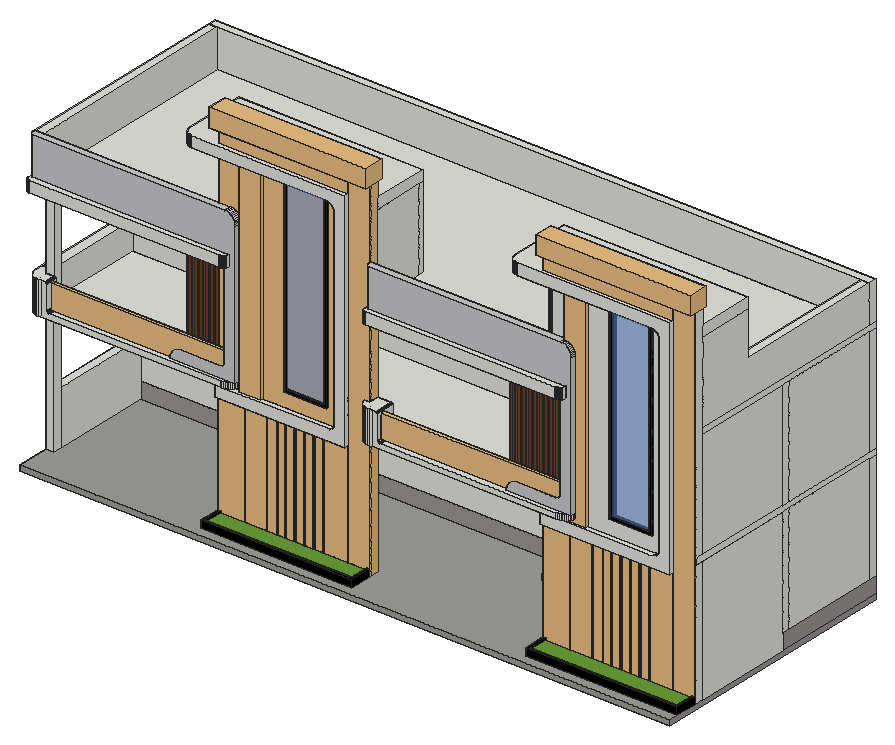
# SketchUp Ruby script. Lengths in inches.
U = 1.inch
M = Sketchup.active_model
def pt(a) = Geom::Point3d.new(a.map { |v| v * U })
def face(e, loops, mat)
  f = e.add_face(loops[0].map { |a| pt(a) })
  loops[1..].each { |l| e.add_face(l.map { |a| pt(a) }).erase! }
  f.material = f.back_material = mat if mat
  f
end
# faces: each face lists its corners as indices into pts; further lists are holes
def faces(e, pts, list, mat = nil) = list.each { |f| face(e, (f[0].is_a?(Array) ? f : [f]).map { |l| l.map { |i| pts[i] } }, mat) }
# xy, xz, yz: faces in a plane at the given z, y or x. An outline is a flat list of corners, or four numbers for a rectangle; further outlines are holes
def ring(l) = l.size == 4 ? [[l[0], l[1]], [l[2], l[1]], [l[2], l[3]], [l[0], l[3]]] : l.each_slice(2).to_a
def flat(e, list, mat, &to3) = list.each { |f| face(e, (f[0].is_a?(Array) ? f : [f]).map { |l| ring(l).map { |u, v| to3.(u, v) } }, mat) }
def xy(e, z, list, mat = nil) = flat(e, list, mat) { |x, y| [x, y, z] }
def xz(e, y, list, mat = nil) = flat(e, list, mat) { |x, z| [x, y, z] }
def yz(e, x, list, mat = nil) = flat(e, list, mat) { |y, z| [x, y, z] }
def lines(e, pts, list) = list.each { |a, b| e.add_line(pt(pts[a]), pt(pts[b])) }
# prism: a flat outline (further loops are holes) pulled along v
def prism(e, loops, v, mat = nil)
  f = face(e, loops, mat); d = Geom::Vector3d.new(v.map { |x| x * U })
  f.pushpull(f.normal.samedirection?(d) ? d.length : -d.length)
end
def box(e, o, s, mat = nil) = prism(e, [[o, [o[0] + s[0], o[1], o[2]], [o[0] + s[0], o[1] + s[1], o[2]], [o[0], o[1] + s[1], o[2]]]], [0, 0, s[2]], mat)
def at(x, y, z, deg = 0) = Geom::Transformation.translation(pt([x, y, z])) * Geom::Transformation.rotation(ORIGIN, Z_AXIS, deg.degrees)
def axes(o, x, y, z) = Geom::Transformation.new([*x, 0, *y, 0, *z, 0, *pt(o).to_a, 1])
def part(name) = M.definitions.add(name)
# library, detail: a bought-in or finely detailed component or shape, given as its bounding box
def library(name, o, s) = part(name).tap { |d| box(d.entities, o, s) }
def detail(e, o, s) = box(e.add_group.entities, o, s)
def put(e, d, t, mat = nil) = e.add_instance(d, t).tap { |i| i.material = mat if mat }
def group(e, t, mat = nil) = e.add_group.tap { |g| g.transformation = t; g.material = mat if mat }.entities
root = M.entities
M.materials.add("[Color M09]").color = [0, 0, 0]
M.materials.add("[Concrete Aggregate Smoke]").color = [154, 150, 148]
M.materials.add("[Concrete Block 8x8 Gray]").color = [157, 158, 154]
M.materials.add("[Grass Dark Green]").color = [106, 157, 55]
M.materials.add("[Polished Concrete New]").color = [200, 200, 203]
M.materials.add("[Translucent Glass Blue]").color = [100, 149, 237]
M.materials["[Translucent Glass Blue]"].alpha = 0.5
M.materials.add("[Wood Bamboo]").color = [177, 105, 43]
M.materials.add("[Wood Cherry Original]").color = [152, 86, 42]
M.materials.add("[Wood Veneer 01]").color = [120, 70, 37]
c1 = part("Group\#3")
prism(c1.entities,[[[0,3,60],[60,3,60],[60,3,0],[0,3,0]],[[27,3,3],[27,3,57],[3,3,57],[3,3,3]],[[33,3,57],[33,3,3],[57,3,3],[57,3,57]]],[0,-3,0])
c2 = part("Group\#4")
xz(c2.entities,0,[[0,0,24,54]])
c3 = part("Group\#5")
xz(c3.entities,0,[[0,0,24,54]])
c4 = part("Group\#6")
prism(c4.entities,[[[60,3,0],[0,3,0],[0,3,60],[60,3,60]],[[57,3,57],[33,3,57],[33,3,3],[57,3,3]],[[3,3,57],[3,3,3],[27,3,3],[27,3,57]]],[0,-3,0])
c5 = part("Group\#7")
xz(c5.entities,0,[[0,0,24,54]])
c6 = part("Group\#8")
xz(c6.entities,0,[[0,0,24,54]])
c7 = part("Group\#9")
prism(c7.entities,[[[3,6,93],[3,6,0],[0,6,0],[0,6,96],[48,6,96],[48,6,0],[45,6,0],[45,6,93]]],[0,-6,0])
c8 = part("Group\#10")
box(c8.entities,[0,0,0],[42,2,93])
c9 = part("Group\#11")
prism(c9.entities,[[[0,1,0.8],[0,1,0],[0,0,0],[0,0,41.3125],[0,1,41.3125],[0,1,40.7],[0,0.3,40.7],[0,0.3,0.8]]],[1.5,0,0])
c10 = part("Group\#12")
prism(c10.entities,[[[3,6,93],[3,6,0],[0,6,0],[0,6,96],[48,6,96],[48,6,0],[45,6,0],[45,6,93]]],[0,-6,0])
c11 = part("Group\#13")
box(c11.entities,[0,0,0],[42,2,93])
c12 = part("Group\#14")
prism(c12.entities,[[[0,1.5,1.15],[0,1.5,0],[0,0,0],[0,0,13.6875],[0,1.5,13.6875],[0,1.5,12.73],[0,0.52,12.73],[0,0.52,1.15]]],[1.4375,0,0])
c13 = part("Group\#16")
box(c13.entities,[0,0,0],[9,111,120])
c14 = part("Group\#17")
box(c14.entities,[0,0,0],[9,111,120])
c15 = library("Group\#20",[0,0,0],[168,9,390])
c16 = library("Group\#22",[0,0,0],[24,2,390])
c17 = library("Group\#23",[0,0,0],[24,2,390])
c18 = part("Group\#30")
box(c18.entities,[0,0,0],[2,1,122])
c19 = part("Group\#31")
put(c19.entities,c18,at(15,0,0))
put(c19.entities,c18,at(48,0,0))
put(c19.entities,c18,at(3,0,0))
put(c19.entities,c18,at(12,0,0))
put(c19.entities,c18,at(33,0,0))
put(c19.entities,c18,at(51,0,0))
put(c19.entities,c18,at(54,0,0))
put(c19.entities,c18,at(39,0,0))
put(c19.entities,c18,at(9,0,0))
put(c19.entities,c18,at(24,0,0))
put(c19.entities,c18,at(18,0,0))
put(c19.entities,c18,at(21,0,0))
put(c19.entities,c18,at(36,0,0))
put(c19.entities,c18,at(30,0,0))
put(c19.entities,c18,at(27,0,0))
put(c19.entities,c18,at(45,0,0))
put(c19.entities,c18,at(42,0,0))
put(c19.entities,c18,at(57,0,0))
put(c19.entities,c18,at(0,0,0))
put(c19.entities,c18,at(6,0,0))
put(c19.entities,c18,at(69,0,0))
put(c19.entities,c18,at(66,0,0))
put(c19.entities,c18,at(63,0,0))
put(c19.entities,c18,at(60,0,0))
c20 = library("Group\#32",[0,0,0],[114,2,122])
c21 = library("Group\#36",[0,0,0],[114,2,122])
c22 = library("Group\#33",[0,0,0],[30,2,122])
c23 = library("Group\#61",[0,0,0],[30,2,122])
c24 = library("Group\#66",[0,0,0],[24,3,226])
c25 = library("Group\#34",[-0.2,0,0],[24.2,3,226])
c26 = library("Group\#44",[0,0,0],[192.84,3.98,26.63])
c27 = library("Group\#62",[0,0,0],[192.84,3.98,26.63])
c28 = library("Group\#52",[-2,0,0],[137,2,18])
c29 = part("Group\#53")
prism(c29.entities,[[[0,33,18],[0,33,0],[0,0,0],[0,0,6],[0,11,6],[0,11,12],[0,22,12],[0,22,18]]],[48,0,0])
c30 = library("Group\#54",[-10.44,-4.48,0],[173.22,22.01,20])
c31 = library("Group\#58",[-9.83,-3.875,0],[172,20.8,20])
c32 = part("Group\#59")
box(c32.entities,[0,0,0],[2.6875,5.375,120])
c33 = part("Group\#60")
put(c33.entities,c32,at(12,0,0))
put(c33.entities,c32,at(0,0,0))
put(c33.entities,c32,at(36,0,0))
put(c33.entities,c32,at(54,0,0))
put(c33.entities,c32,at(48,0,0))
put(c33.entities,c32,at(30,0,0))
put(c33.entities,c32,at(6,0,0))
put(c33.entities,c32,at(24,0,0))
put(c33.entities,c32,at(18,0,0))
put(c33.entities,c32,at(42,0,0))
c34 = part("Group\#65")
xy(c34.entities,0,[[0,0,168,24]])
xy(c34.entities,6.3125,[[3,3,165,24]],"[Grass Dark Green]")
xy(c34.entities,8,[[0,0,168,0,168,24,165,24,165,3,3,3,3,24,0,24]])
xz(c34.entities,0,[[0,0,168,8]])
xz(c34.entities,3,[[3,6.3125,165,8]])
xz(c34.entities,24,[[0,0,0,8,3,8,3,6.3125,165,6.3125,165,8,168,8,168,0]])
yz(c34.entities,0,[[0,0,24,8]])
yz(c34.entities,3,[[3,6.3125,24,8]])
yz(c34.entities,165,[[3,6.3125,24,8]])
yz(c34.entities,168,[[0,0,24,8]])
box(root,[276.07,44.3,150],[48,0.7,210])
box(root,[636.07,44.4,150],[48,0.6,210])
xy(root,138,[[590.07,35,600.07,35,588.38,35.84]])
p = [[586.19,36,138],[588.38,35.84,138],[588.07,36,138],[366.35,34,138],[366.35,34,174],[372.07,34,174],
  [372.07,45,174],[215.75,27.83,270],[221.82,27.83,270],[221.82,27.83,257.98],[593.94,27.83,270],[588.07,27.83,270],
  [593.94,27.83,258.125],[593.94,27.83,257.98],[588.07,27.83,257.98],[207.03,39.48,360],[206.71,40.1,360],[206.39,40.72,360],
  [206.07,41.34,360],[205.74,41.95,360],[205.41,42.5625,360],[205.08,43.18,360],[204.74,43.79,360],[204.07,45,360],
  [204.41,44.39,360],[207.34,38.86,360],[207.65,38.24,360],[207.96,37.61,360]]
lines(root,p,[[0,1],[1,2],[3,4],[4,5],[5,6],[7,8],[8,9],[10,11],[10,12],[12,13],[13,14],[15,16],
  [16,17],[17,18],[18,19],[19,20],[20,21],[21,22],[23,24],[24,22],[15,25],[25,26],[26,27]])
g1 = group(root,at(12.07,45,6),"[Concrete Aggregate Smoke]")
xy(g1,-12,[[0,-45,720,240]])
xy(g1,-6,[[0,111,720,240]])
xy(g1,-6,[[0,-45,720,111]],"[Concrete Block 8x8 Gray]")
xy(g1,12,[[0,111,720,240]])
xz(g1,-45,[[0,-12,720,-6]],"[Concrete Block 8x8 Gray]")
xz(g1,111,[[0,-6,720,12]])
xz(g1,240,[[0,-12,720,-6],[0,-6,720,12]])
yz(g1,0,[[-45,-12,240,-6],[111,-6,240,12]])
yz(g1,720,[[-45,-12,240,-6],[111,-6,240,12]])
g2 = group(root,at(12.07,156,18))
prism(g2,[[[720,9,0],[528,9,0],[528,9,96],[480,9,96],[480,9,0],[180,9,0],[180,9,96],[132,9,96],[132,9,0],[0,9,0],[0,9,120],[720,9,120]],[[36,9,96],[36,9,36],[96,9,36],[96,9,96]],[[444,9,36],[444,9,96],[384,9,96],[384,9,36]]],[0,-9,0])
put(root,c1,at(48.07,156,54),"[Wood Veneer 01]")
put(root,c2,at(81.07,156,57),"[Translucent Glass Blue]")
put(root,c3,at(51.07,156,57),"[Translucent Glass Blue]")
put(root,c4,at(396.07,156,54),"[Wood Veneer 01]")
put(root,c5,at(429.07,156,57),"[Translucent Glass Blue]")
put(root,c6,at(399.07,156,57),"[Translucent Glass Blue]")
put(root,c7,at(144.07,156,18),"[Wood Bamboo]")
put(root,c8,at(147.07,159,18),"[Wood Bamboo]")
put(root,c9,at(151.76,158,35.81),"[Wood Bamboo]")
put(root,c10,at(492.07,156,18),"[Wood Bamboo]")
put(root,c11,at(495.07,159,18),"[Wood Bamboo]")
put(root,c12,at(497.5625,157.5,63.91),"[Wood Bamboo]")
g3 = group(root,at(12.07,276,18))
box(g3,[0,0,0],[720,9,120])
put(root,c13,at(12.07,165,18))
put(root,c14,at(723.07,165,18))
put(root,c8,at(147.07,159,144),"[Wood Bamboo]")
g4 = group(root,at(12.07,276,144))
box(g4,[-11.67,0,0],[731.67,9,120])
put(root,c12,at(497.5625,157.5,189.91),"[Wood Bamboo]")
put(root,c7,at(144.07,156,144),"[Wood Bamboo]")
put(root,c1,at(48.07,156,180),"[Wood Veneer 01]")
put(root,c13,at(0.39,165,144))
put(root,c11,at(495.07,159,144),"[Wood Bamboo]")
put(root,c2,at(81.07,156,183),"[Translucent Glass Blue]")
put(root,c5,at(429.07,156,183),"[Translucent Glass Blue]")
put(root,c3,at(51.07,156,183),"[Translucent Glass Blue]")
put(root,c4,at(396.07,156,180),"[Wood Veneer 01]")
put(root,c6,at(399.07,156,183),"[Translucent Glass Blue]")
put(root,c14,at(723.07,165,144))
put(root,c10,at(492.07,156,144),"[Wood Bamboo]")
g5 = group(root,at(12.07,156,144))
prism(g5,[[[720,9,0],[528,9,0],[528,9,96],[480,9,96],[480,9,0],[180,9,0],[180,9,96],[132,9,96],[132,9,0],[-11.67,9,0],[-11.67,9,120],[720,9,120]],[[36,9,96],[36,9,36],[96,9,36],[96,9,96]],[[444,9,36],[444,9,96],[384,9,96],[384,9,36]]],[0,-9,0])
put(root,c9,at(151.76,158,161.81),"[Wood Bamboo]")
g6 = group(root,at(12.07,156,138))
prism(g6,[[[720,129,0],[720,-119.45,0],[9,-119.45,0],[9,-111,0],[-11.67,-111,0],[-11.67,0,0],[-11.67,129,0]]],[0,0,6])
g7 = group(root,at(12.07,36,0))
prism(g7,[[[9,0,0],[9,9,0],[9,9,264],[9,0.55,264],[9,0.55,138],[9,0,138]]],[-9,0,0])
put(root,c15,at(204.07,36,0))
g8 = group(root,at(564.07,36,0))
xy(g8,0,[[0,0,168,9]])
xy(g8,138,[[0,0,22.125,9]])
xy(g8,150,[[72,0,120,9]])
xy(g8,264,[[9,0,7.83,0.08,6.67,0.31,5.56,0.69,4.5,1.21,3.52,1.86,2.64,2.64,1.86,3.52,1.21,4.5,0.69,5.56,0.31,6.67,0.08,7.83,0,9,22.125,9,22.125,0]])
xy(g8,360,[[72,0,120,9]])
xy(g8,390,[[9,0,168,0,168,9,0,9,0.08,7.83,0.31,6.67,0.69,5.56,1.21,4.5,1.86,3.52,2.64,2.64,3.52,1.86,4.5,1.21,5.56,0.69,6.67,0.31,7.83,0.08]])
xz(g8,0,[[[0,0,168,0,168,390,9,390,9,264,22.125,264,22.125,138,0,138],[72,150,120,360]]])
xz(g8,9,[[[0,0,0,138,22.125,138,22.125,264,0,264,0,390,168,390,168,0],[72,150,120,360]]])
yz(g8,0,[[0,0,9,138]])
yz(g8,22.125,[[0,138,9,264]])
yz(g8,72,[[0,150,9,360]])
yz(g8,120,[[0,150,9,360]])
yz(g8,168,[[0,0,9,390]])
p = [[9,0,390],[7.83,0.08,390],[7.83,0.08,264],[9,0,264],[6.67,0.31,390],[6.67,0.31,264],
  [5.56,0.69,390],[5.56,0.69,264],[4.5,1.21,390],[4.5,1.21,264],[3.52,1.86,390],[3.52,1.86,264],
  [2.64,2.64,390],[2.64,2.64,264],[1.86,3.52,390],[1.86,3.52,264],[1.21,4.5,390],[1.21,4.5,264],
  [0.69,5.56,390],[0.69,5.56,264],[0.31,6.67,390],[0.31,6.67,264],[0.08,7.83,390],[0.08,7.83,264],
  [0,9,390],[0,9,264]]
faces(g8,p,[[0,1,2,3],[1,4,5,2],[4,6,7,5],[6,8,9,7],[8,10,11,9],[10,12,13,11],[12,14,15,13],[14,16,17,15],
  [16,18,19,17],[18,20,21,19],[20,22,23,21],[22,24,25,23]])
put(root,c16,at(348.07,34,0),"[Polished Concrete New]")
put(root,c17,at(708.07,34,0),"[Polished Concrete New]")
g9 = group(root,at(204.07,30,122))
xy(g9,0,[[0,0,144,6]])
xy(g9,12,[[11.49,0,126.92,6]])
xy(g9,16,[[0,0,11.49,6]])
xy(g9,238,[[-25.46,0,-26.83,0.09,-28.1875,0.36,-29.49,0.8,-30.73,1.41,-31.875,2.18,-32.91,3.09,-33.82,4.125,-34.59,5.27,-35.2,6.51,-35.64,7.8125,-35.91,9.17,-36,10.54,-36,78,168,78,168,15,3.89,15,3.89,6,122.55,6,122.55,0]])
xy(g9,250,[[-25.46,0,144,0,144,6,3.89,6,3.89,15,168,15,168,78,-36,78,-36,10.54,-35.91,9.17,-35.64,7.8125,-35.2,6.51,-34.59,5.27,-33.82,4.125,-32.91,3.09,-31.875,2.18,-30.73,1.41,-29.49,0.8,-28.1875,0.36,-26.83,0.09]])
xz(g9,0,[[0,0,144,0,144,250,-25.46,250,-25.46,238,122.55,238,123.78,237.92,124.99,237.68,126.17,237.28,127.27,236.73,128.3,236.05,129.23,235.23,130.05,234.3,130.73,233.27,131.28,232.17,131.68,230.99,131.92,229.78,132,228.55,132,17.08,131.96,16.42,131.83,15.77,131.61,15.14,131.32,14.54,130.95,13.99,130.51,13.49,130.01,13.05,129.46,12.68,128.86,12.39,128.23,12.17,127.58,12.04,126.92,12,11.49,12,11.49,16,0,16]])
xz(g9,6,[[0,0,0,16,11.49,16,11.49,12,126.92,12,127.58,12.04,128.23,12.17,128.86,12.39,129.46,12.68,130.01,13.05,130.51,13.49,130.95,13.99,131.32,14.54,131.61,15.14,131.83,15.77,131.96,16.42,132,17.08,132,228.55,131.92,229.78,131.68,230.99,131.28,232.17,130.73,233.27,130.05,234.3,129.23,235.23,128.3,236.05,127.27,236.73,126.17,237.28,124.99,237.68,123.78,237.92,122.55,238,3.89,238,3.89,250,144,250,144,0]])
xz(g9,15,[[3.89,238,168,250]])
xz(g9,78,[[-36,238,168,250]])
yz(g9,-36,[[10.54,238,78,250]])
yz(g9,0,[[0,0,6,16]])
yz(g9,3.89,[[6,238,15,250]])
yz(g9,11.49,[[0,12,6,16]])
yz(g9,132,[[0,17.08,6,228.55]])
yz(g9,144,[[0,0,6,250]])
yz(g9,168,[[15,238,78,250]])
p = [[127.58,6,12.04],[126.92,6,12],[126.92,0,12],[127.58,0,12.04],[128.23,6,12.17],[128.23,0,12.17],
  [128.86,6,12.39],[128.86,0,12.39],[129.46,6,12.68],[129.46,0,12.68],[130.01,6,13.05],[130.01,0,13.05],
  [130.51,6,13.49],[130.51,0,13.49],[130.95,6,13.99],[130.95,0,13.99],[131.32,6,14.54],[131.32,0,14.54],
  [131.61,6,15.14],[131.61,0,15.14],[131.83,6,15.77],[131.83,0,15.77],[131.96,6,16.42],[131.96,0,16.42],
  [132,6,17.08],[132,0,17.08],[131.92,6,229.78],[132,6,228.55],[132,0,228.55],[131.92,0,229.78],
  [131.68,6,230.99],[131.68,0,230.99],[131.28,6,232.17],[131.28,0,232.17],[130.73,6,233.27],[130.73,0,233.27],
  [130.05,6,234.3],[130.05,0,234.3],[129.23,6,235.23],[129.23,0,235.23],[128.3,6,236.05],[128.3,0,236.05],
  [127.27,6,236.73],[127.27,0,236.73],[126.17,6,237.28],[126.17,0,237.28],[124.99,6,237.68],[124.99,0,237.68],
  [123.78,6,237.92],[123.78,0,237.92],[122.55,6,238],[122.55,0,238],[-25.46,0,250],[-26.83,0.09,250],
  [-26.83,0.09,238],[-25.46,0,238],[-28.1875,0.36,250],[-28.1875,0.36,238],[-29.49,0.8,250],[-29.49,0.8,238],
  [-30.73,1.41,250],[-30.73,1.41,238],[-31.875,2.18,250],[-31.875,2.18,238],[-32.91,3.09,250],[-32.91,3.09,238],
  [-33.82,4.125,250],[-33.82,4.125,238],[-34.59,5.27,250],[-34.59,5.27,238],[-35.2,6.51,250],[-35.2,6.51,238],
  [-35.64,7.8125,250],[-35.64,7.8125,238],[-35.91,9.17,250],[-35.91,9.17,238],[-36,10.54,250],[-36,10.54,238]]
faces(g9,p,[[0,1,2,3],[4,0,3,5],[6,4,5,7],[8,6,7,9],[10,8,9,11],[12,10,11,13],[14,12,13,15],[16,14,15,17],
  [18,16,17,19],[20,18,19,21],[22,20,21,23],[24,22,23,25],[26,27,28,29],[30,26,29,31],[32,30,31,33],[34,32,33,35],
  [36,34,35,37],[38,36,37,39],[40,38,39,41],[42,40,41,43],[44,42,43,45],[46,44,45,47],[48,46,47,49],[50,48,49,51],
  [52,53,54,55],[53,56,57,54],[56,58,59,57],[58,60,61,59],[60,62,63,61],[62,64,65,63],[64,66,67,65],[66,68,69,67],
  [68,70,71,69],[70,72,73,71],[72,74,75,73],[74,76,77,75]])
g10 = group(root,at(564.07,30,122))
xy(g10,0,[[0,0,144,6]])
xy(g10,12,[[11.8,0,124.1,6]])
xy(g10,16,[[0,0,11.8,6]])
xy(g10,238,[[-24.32,0,-25.84,0.1,-27.34,0.4,-28.79,0.89,-30.16,1.57,-31.43,2.41,-32.58,3.42,-33.59,4.57,-34.43,5.84,-35.11,7.21,-35.6,8.66,-35.9,10.16,-36,11.68,-36,78,168,78,168,15,2.79,15,2.79,6,123.21,6,123.21,0]])
xy(g10,250,[[-24.32,0,144,0,144,6,2.79,6,2.79,15,168,15,168,78,-36,78,-36,11.68,-35.9,10.16,-35.6,8.66,-35.11,7.21,-34.43,5.84,-33.59,4.57,-32.58,3.42,-31.43,2.41,-30.16,1.57,-28.79,0.89,-27.34,0.4,-25.84,0.1]])
xz(g10,0,[[0,0,144,0,144,250,-24.32,250,-24.32,238,123.21,238,124.36,237.92,125.49,237.7,126.58,237.33,127.61,236.82,128.5625,236.18,129.43,235.43,130.18,234.5625,130.82,233.61,131.33,232.58,131.7,231.49,131.92,230.36,132,229.21,132,19.9,131.93,18.87,131.73,17.86,131.4,16.88,130.94,15.95,130.37,15.09,129.6875,14.3125,128.91,13.63,128.05,13.06,127.12,12.6,126.14,12.27,125.13,12.07,124.1,12,11.8,12,11.8,16,0,16]])
xz(g10,6,[[0,0,0,16,11.8,16,11.8,12,124.1,12,125.13,12.07,126.14,12.27,127.12,12.6,128.05,13.06,128.91,13.63,129.6875,14.3125,130.37,15.09,130.94,15.95,131.4,16.88,131.73,17.86,131.93,18.87,132,19.9,132,229.21,131.92,230.36,131.7,231.49,131.33,232.58,130.82,233.61,130.18,234.5625,129.43,235.43,128.5625,236.18,127.61,236.82,126.58,237.33,125.49,237.7,124.36,237.92,123.21,238,2.79,238,2.79,250,144,250,144,0]])
xz(g10,15,[[2.79,238,168,250]])
xz(g10,78,[[-36,238,168,250]])
yz(g10,-36,[[11.68,238,78,250]])
yz(g10,0,[[0,0,6,16]])
yz(g10,2.79,[[6,238,15,250]])
yz(g10,11.8,[[0,12,6,16]])
yz(g10,132,[[0,19.9,6,229.21]])
yz(g10,144,[[0,0,6,250]])
yz(g10,168,[[15,238,78,250]])
p = [[125.13,6,12.07],[124.1,6,12],[124.1,0,12],[125.13,0,12.07],[126.14,6,12.27],[126.14,0,12.27],
  [127.12,6,12.6],[127.12,0,12.6],[128.05,6,13.06],[128.05,0,13.06],[128.91,6,13.63],[128.91,0,13.63],
  [129.6875,6,14.3125],[129.6875,0,14.3125],[130.37,6,15.09],[130.37,0,15.09],[130.94,6,15.95],[130.94,0,15.95],
  [131.4,6,16.88],[131.4,0,16.88],[131.73,6,17.86],[131.73,0,17.86],[131.93,6,18.87],[131.93,0,18.87],
  [132,6,19.9],[132,0,19.9],[131.92,6,230.36],[132,6,229.21],[132,0,229.21],[131.92,0,230.36],
  [131.7,6,231.49],[131.7,0,231.49],[131.33,6,232.58],[131.33,0,232.58],[130.82,6,233.61],[130.82,0,233.61],
  [130.18,6,234.5625],[130.18,0,234.5625],[129.43,6,235.43],[129.43,0,235.43],[128.5625,6,236.18],[128.5625,0,236.18],
  [127.61,6,236.82],[127.61,0,236.82],[126.58,6,237.33],[126.58,0,237.33],[125.49,6,237.7],[125.49,0,237.7],
  [124.36,6,237.92],[124.36,0,237.92],[123.21,6,238],[123.21,0,238],[-24.32,0,250],[-25.84,0.1,250],
  [-25.84,0.1,238],[-24.32,0,238],[-27.34,0.4,250],[-27.34,0.4,238],[-28.79,0.89,250],[-28.79,0.89,238],
  [-30.16,1.57,250],[-30.16,1.57,238],[-31.43,2.41,250],[-31.43,2.41,238],[-32.58,3.42,250],[-32.58,3.42,238],
  [-33.59,4.57,250],[-33.59,4.57,238],[-34.43,5.84,250],[-34.43,5.84,238],[-35.11,7.21,250],[-35.11,7.21,238],
  [-35.6,8.66,250],[-35.6,8.66,238],[-35.9,10.16,250],[-35.9,10.16,238],[-36,11.68,250],[-36,11.68,238]]
faces(g10,p,[[0,1,2,3],[4,0,3,5],[6,4,5,7],[8,6,7,9],[10,8,9,11],[12,10,11,13],[14,12,13,15],[16,14,15,17],
  [18,16,17,19],[20,18,19,21],[22,20,21,23],[24,22,23,25],[26,27,28,29],[30,26,29,31],[32,30,31,33],[34,32,33,35],
  [36,34,35,37],[38,36,37,39],[40,38,39,41],[42,40,41,43],[44,42,43,45],[46,44,45,47],[48,46,47,49],[50,48,49,51],
  [52,53,54,55],[53,56,57,54],[56,58,59,57],[58,60,61,59],[60,62,63,61],[62,64,65,63],[64,66,67,65],[66,68,69,67],
  [68,70,71,69],[70,72,73,71],[72,74,75,73],[74,76,77,75]])
g11 = group(root,at(276.07,35,150),"[Color M09]")
prism(g11,[[[0,4,0],[0,4,210],[48,4,210],[48,4,0]],[[45,4,207],[3,4,207],[3,4,3],[45,4,3]]],[0,-4,0])
g12 = group(root,at(279.07,36,153),"[Translucent Glass Blue]")
xz(g12,0,[[0,0,42,204]])
g13 = group(root,at(636.07,35,150))
prism(g13,[[[0,4,0],[0,4,210],[48,4,210],[48,4,0]],[[3,4,3],[45,4,3],[45,4,207],[3,4,207]]],[0,-4,0],"[Color M09]")
g14 = group(root,at(639.07,36,153),"[Translucent Glass Blue]")
xz(g14,0,[[0,0,42,204]])
put(root,c19,at(252.07,35,0),"[Wood Bamboo]")
put(root,c20,at(234.07,34,0))
put(root,c19,at(613.07,35,0),"[Wood Bamboo]")
put(root,c21,at(594.07,34,0))
put(root,c22,at(204.07,34,0))
put(root,c23,at(564.07,34,0))
put(root,c24,at(228.07,33,134),"[Wood Cherry Original]")
put(root,c25,at(588.07,33,134),"[Wood Cherry Original]")
g15 = group(root,at(16.39,24,138))
xy(g15,0,[[-3.89,-0.41,-5.81,-0.17,-7.67,0.37,-9.43,1.19,-11.05,2.28,-12.48,3.6,-12.88,4.09,-4.23,4.09,-4.2,3.61,-4.1,3.125,-3.93,2.66,-3.69,2.21,-3.4,1.79,-3.05,1.4,-2.64,1.05,-2.19,0.74,-1.7,0.48,-1.17,0.26,-0.625,0.1,-0.05,0,-1.96,-0.35],[-0.05,0,-0.625,0.1,-1.17,0.26,-1.7,0.48,-2.19,0.74,-2.64,1.05,-3.05,1.4,-3.4,1.79,-3.69,2.21,-3.93,2.66,-4.1,3.125,-4.2,3.61,-4.23,4.09,-12.88,4.09,-13.71,5.125,-14.69,6.82,-15.41,8.66,-15.85,10.58,-15.99,12.55,-15.99,21,-4.32,21,-4.32,12.55,211.68,12.55,211.68,10.85,211.57,9.4375,211.24,8.04,210.69,6.7,209.94,5.43,209,4.25,207.88,3.18,206.6,2.24,205.19,1.45,203.67,0.83,202.0625,0.37,200.4,0.09,198.7,0]])
xy(g15,6,[[9.74,0,198.7,0,200.4,0.09,202.0625,0.37,203.67,0.83,205.19,1.45,206.6,2.24,207.88,3.18,209,4.25,209.94,5.43,210.69,6.7,211.24,8.04,211.57,9.4375,211.68,10.85,211.68,12.55,9.74,12.55]])
xy(g15,36,[[-3.89,-0.41,-1.96,-0.35,-0.05,0,4.125,0,4.125,12.55,-4.32,12.55,-4.32,21,-15.99,21,-15.99,12.55,-15.85,10.58,-15.41,8.66,-14.69,6.82,-13.71,5.125,-12.88,4.09,-12.48,3.6,-11.05,2.28,-9.43,1.19,-7.67,0.37,-5.81,-0.17]])
xz(g15,0,[[-0.05,0,198.7,0,198.7,6,9.74,6,9.32,6.02,8.91,6.09,8.51,6.2,8.13,6.36,7.78,6.55,7.47,6.79,7.19,7.05,6.96,7.34,6.77,7.66,6.64,7.99,6.56,8.33,6.53,8.68,6.53,33.99,6.51,34.25,6.45,34.51,6.35,34.76,6.21,35,6.03,35.21,5.82,35.41,5.59,35.58,5.33,35.73,5.05,35.85,4.75,35.93,4.4375,35.98,4.125,36,-0.05,36]])
xz(g15,12.55,[[-4.32,0,-4.32,36,4.125,36,4.4375,35.98,4.75,35.93,5.05,35.85,5.33,35.73,5.59,35.58,5.82,35.41,6.03,35.21,6.21,35,6.35,34.76,6.45,34.51,6.51,34.25,6.53,33.99,6.53,8.68,6.56,8.33,6.64,7.99,6.77,7.66,6.96,7.34,7.19,7.05,7.47,6.79,7.78,6.55,8.13,6.36,8.51,6.2,8.91,6.09,9.32,6.02,9.74,6,211.68,6,211.68,0]])
xz(g15,21,[[-15.99,0,-4.32,36]])
yz(g15,-15.99,[[12.55,0,21,36]])
yz(g15,-4.32,[[12.55,0,21,36]])
yz(g15,6.53,[[0,8.68,12.55,33.99]])
yz(g15,211.68,[[10.85,0,12.55,6]])
p = [[-3.89,-0.41,36],[-5.81,-0.17,36],[-5.81,-0.17,0],[-3.89,-0.41,0],[-1.96,-0.35,36],[-1.96,-0.35,0],
  [-0.05,0,36],[-0.05,0,0],[-7.67,0.37,36],[-7.67,0.37,0],[200.4,0.09,6],[198.7,0,6],
  [198.7,0,0],[200.4,0.09,0],[202.0625,0.37,6],[202.0625,0.37,0],[-9.43,1.19,36],[-9.43,1.19,0],
  [203.67,0.83,6],[203.67,0.83,0],[205.19,1.45,6],[205.19,1.45,0],[-11.05,2.28,36],[-11.05,2.28,0],
  [206.6,2.24,6],[206.6,2.24,0],[207.88,3.18,6],[207.88,3.18,0],[-12.48,3.6,36],[-12.48,3.6,0],
  [209,4.25,6],[209,4.25,0],[-12.88,4.09,36],[-12.88,4.09,0],[-13.71,5.125,36],[-13.71,5.125,0],
  [209.94,5.43,6],[209.94,5.43,0],[-14.69,6.82,36],[-14.69,6.82,0],[210.69,6.7,6],[210.69,6.7,0],
  [211.24,8.04,6],[211.24,8.04,0],[-15.41,8.66,36],[-15.41,8.66,0],[211.57,9.4375,6],[211.57,9.4375,0],
  [-15.85,10.58,36],[-15.85,10.58,0],[211.68,10.85,6],[211.68,10.85,0],[-15.99,12.55,36],[-15.99,12.55,0],
  [9.32,12.55,6.02],[8.91,12.55,6.09],[8.91,0,6.09],[9.32,0,6.02],[9.74,12.55,6],[9.74,0,6],
  [8.51,12.55,6.2],[8.51,0,6.2],[8.13,12.55,6.36],[8.13,0,6.36],[7.78,12.55,6.55],[7.78,0,6.55],
  [7.47,12.55,6.79],[7.47,0,6.79],[7.19,12.55,7.05],[7.19,0,7.05],[6.96,12.55,7.34],[6.96,0,7.34],
  [6.77,12.55,7.66],[6.77,0,7.66],[6.64,12.55,7.99],[6.64,0,7.99],[6.56,12.55,8.33],[6.56,0,8.33],
  [6.53,12.55,8.68],[6.53,0,8.68],[6.53,12.55,33.99],[6.51,12.55,34.25],[6.51,0,34.25],[6.53,0,33.99],
  [6.45,12.55,34.51],[6.45,0,34.51],[6.35,12.55,34.76],[6.35,0,34.76],[6.21,12.55,35],[6.21,0,35],
  [6.03,12.55,35.21],[6.03,0,35.21],[5.82,12.55,35.41],[5.82,0,35.41],[5.59,12.55,35.58],[5.59,0,35.58],
  [5.33,12.55,35.73],[5.33,0,35.73],[5.05,12.55,35.85],[5.05,0,35.85],[4.75,12.55,35.93],[4.75,0,35.93],
  [4.4375,12.55,35.98],[4.4375,0,35.98],[4.125,12.55,36],[4.125,0,36],[-4.1,3.125,33.15],[-4.23,4.09,36],
  [-4.23,4.09,0]]
faces(g15,p,[[0,1,2,3],[4,0,3,5],[6,4,5,7],[1,8,9,2],[10,11,12,13],[14,10,13,15],[8,16,17,9],[18,14,15,19],
  [20,18,19,21],[16,22,23,17],[24,20,21,25],[26,24,25,27],[22,28,29,23],[30,26,27,31],[28,32,33,29],[32,34,35,33],
  [36,30,31,37],[34,38,39,35],[40,36,37,41],[42,40,41,43],[38,44,45,39],[46,42,43,47],[44,48,49,45],[50,46,47,51],
  [48,52,53,49],[54,55,56,57],[58,54,57,59],[55,60,61,56],[60,62,63,61],[62,64,65,63],[64,66,67,65],[66,68,69,67],
  [68,70,71,69],[70,72,73,71],[72,74,75,73],[74,76,77,75],[76,78,79,77],[80,81,82,83],[81,84,85,82],[84,86,87,85],
  [86,88,89,87],[88,90,91,89],[90,92,93,91],[92,94,95,93],[94,96,97,95],[96,98,99,97],[98,100,101,99],[100,102,103,101],
  [102,104,105,103]])
lines(g15,p,[[106,6],[107,108]])
g16 = group(root,at(382.51,24,138))
xy(g16,0,[[-4,-0.41,-5.97,-0.17,-7.89,0.37,-9.7,1.19,-11.36,2.28,-12.84,3.6,-13.25,4.09,-4.35,4.09,-4.32,3.61,-4.21,3.125,-4.04,2.66,-3.8,2.21,-3.5,1.79,-3.13,1.4,-2.72,1.05,-2.25,0.74,-1.75,0.48,-1.21,0.26,-0.64,0.1,-0.06,0,-2.01,-0.35],[-0.06,0,-0.64,0.1,-1.21,0.26,-1.75,0.48,-2.25,0.74,-2.72,1.05,-3.13,1.4,-3.5,1.79,-3.8,2.21,-4.04,2.66,-4.21,3.125,-4.32,3.61,-4.35,4.09,-13.25,4.09,-14.1,5.125,-15.11,6.82,-15.85,8.66,-16.3,10.58,-16.45,12.55,-16.45,21,217.73,21,217.73,10.85,217.61,9.4375,217.27,8.04,216.71,6.7,215.94,5.43,214.97,4.25,213.82,3.18,212.51,2.24,211.05,1.45,209.49,0.83,207.83,0.37,206.12,0.09,204.38,0]])
xy(g16,6,[[10.01,0,204.38,0,206.12,0.09,207.83,0.37,209.49,0.83,211.05,1.45,212.51,2.24,213.82,3.18,214.97,4.25,215.94,5.43,216.71,6.7,217.27,8.04,217.61,9.4375,217.73,10.85,217.73,21,10.01,21]])
xy(g16,36,[[-4,-0.41,-2.01,-0.35,-0.06,0,4.24,0,4.24,21,-16.45,21,-16.45,12.55,-16.3,10.58,-15.85,8.66,-15.11,6.82,-14.1,5.125,-13.25,4.09,-12.84,3.6,-11.36,2.28,-9.7,1.19,-7.89,0.37,-5.97,-0.17]])
xz(g16,0,[[-0.06,0,204.38,0,204.38,6,10.01,6,9.58,6.02,9.16,6.09,8.75,6.2,8.36,6.36,8.01,6.55,7.68,6.79,7.4,7.05,7.16,7.34,6.97,7.66,6.83,7.99,6.74,8.33,6.71,8.68,6.71,33.99,6.69,34.25,6.63,34.51,6.53,34.76,6.38,35,6.2,35.21,5.99,35.41,5.75,35.58,5.48,35.73,5.1875,35.85,4.88,35.93,4.57,35.98,4.24,36,-0.06,36]])
xz(g16,21,[[-16.45,0,-16.45,36,4.24,36,4.57,35.98,4.88,35.93,5.1875,35.85,5.48,35.73,5.75,35.58,5.99,35.41,6.2,35.21,6.38,35,6.53,34.76,6.63,34.51,6.69,34.25,6.71,33.99,6.71,8.68,6.74,8.33,6.83,7.99,6.97,7.66,7.16,7.34,7.4,7.05,7.68,6.79,8.01,6.55,8.36,6.36,8.75,6.2,9.16,6.09,9.58,6.02,10.01,6,217.73,6,217.73,0]])
yz(g16,-16.45,[[12.55,0,21,36]])
yz(g16,6.71,[[0,8.68,21,33.99]])
yz(g16,217.73,[[10.85,0,21,6]])
p = [[-4,-0.41,36],[-5.97,-0.17,36],[-5.97,-0.17,0],[-4,-0.41,0],[-2.01,-0.35,36],[-2.01,-0.35,0],
  [-0.06,0,36],[-0.06,0,0],[-7.89,0.37,36],[-7.89,0.37,0],[206.12,0.09,6],[204.38,0,6],
  [204.38,0,0],[206.12,0.09,0],[207.83,0.37,6],[207.83,0.37,0],[-9.7,1.19,36],[-9.7,1.19,0],
  [209.49,0.83,6],[209.49,0.83,0],[211.05,1.45,6],[211.05,1.45,0],[-11.36,2.28,36],[-11.36,2.28,0],
  [212.51,2.24,6],[212.51,2.24,0],[213.82,3.18,6],[213.82,3.18,0],[-12.84,3.6,36],[-12.84,3.6,0],
  [214.97,4.25,6],[214.97,4.25,0],[-13.25,4.09,36],[-13.25,4.09,0],[-14.1,5.125,36],[-14.1,5.125,0],
  [215.94,5.43,6],[215.94,5.43,0],[-15.11,6.82,36],[-15.11,6.82,0],[216.71,6.7,6],[216.71,6.7,0],
  [217.27,8.04,6],[217.27,8.04,0],[-15.85,8.66,36],[-15.85,8.66,0],[217.61,9.4375,6],[217.61,9.4375,0],
  [-16.3,10.58,36],[-16.3,10.58,0],[217.73,10.85,6],[217.73,10.85,0],[-16.45,12.55,36],[-16.45,12.55,0],
  [9.58,21,6.02],[9.16,21,6.09],[9.16,0,6.09],[9.58,0,6.02],[10.01,21,6],[10.01,0,6],
  [8.75,21,6.2],[8.75,0,6.2],[8.36,21,6.36],[8.36,0,6.36],[8.01,21,6.55],[8.01,0,6.55],
  [7.68,21,6.79],[7.68,0,6.79],[7.4,21,7.05],[7.4,0,7.05],[7.16,21,7.34],[7.16,0,7.34],
  [6.97,21,7.66],[6.97,0,7.66],[6.83,21,7.99],[6.83,0,7.99],[6.74,21,8.33],[6.74,0,8.33],
  [6.71,21,8.68],[6.71,0,8.68],[6.71,21,33.99],[6.69,21,34.25],[6.69,0,34.25],[6.71,0,33.99],
  [6.63,21,34.51],[6.63,0,34.51],[6.53,21,34.76],[6.53,0,34.76],[6.38,21,35],[6.38,0,35],
  [6.2,21,35.21],[6.2,0,35.21],[5.99,21,35.41],[5.99,0,35.41],[5.75,21,35.58],[5.75,0,35.58],
  [5.48,21,35.73],[5.48,0,35.73],[5.1875,21,35.85],[5.1875,0,35.85],[4.88,21,35.93],[4.88,0,35.93],
  [4.57,21,35.98],[4.57,0,35.98],[4.24,21,36],[4.24,0,36],[-4.21,3.125,33.15],[-4.35,4.09,36],
  [-4.35,4.09,0]]
faces(g16,p,[[0,1,2,3],[4,0,3,5],[6,4,5,7],[1,8,9,2],[10,11,12,13],[14,10,13,15],[8,16,17,9],[18,14,15,19],
  [20,18,19,21],[16,22,23,17],[24,20,21,25],[26,24,25,27],[22,28,29,23],[30,26,27,31],[28,32,33,29],[32,34,35,33],
  [36,30,31,37],[34,38,39,35],[40,36,37,41],[42,40,41,43],[38,44,45,39],[46,42,43,47],[44,48,49,45],[50,46,47,51],
  [48,52,53,49],[54,55,56,57],[58,54,57,59],[55,60,61,56],[60,62,63,61],[62,64,65,63],[64,66,67,65],[66,68,69,67],
  [68,70,71,69],[70,72,73,71],[72,74,75,73],[74,76,77,75],[76,78,79,77],[80,81,82,83],[81,84,85,82],[84,86,87,85],
  [86,88,89,87],[88,90,91,89],[90,92,93,91],[92,94,95,93],[94,96,97,95],[96,98,99,97],[98,100,101,99],[100,102,103,101],
  [102,104,105,103]])
lines(g16,p,[[106,6],[107,108]])
g17 = group(root,at(372.3125,27.83,144),"[Polished Concrete New]")
xy(g17,0,[[155.75,0,215.75,8.17],[215.75,0,217.75,8.17],[217.75,0,228,8.17]])
xy(g17,12,[[167.75,0,211.64,8.17]])
xy(g17,126,[[3.78,0,3.23,0.29,2.71,0.64,2.23,1.03,1.78,1.46,1.38,1.9375,1.02,2.45,0.72,2.99,0.46,3.56,0.26,4.15,0.12,4.75,0.03,5.37,0,5.99,0,8.17,215.75,8.17,215.75,0]])
xy(g17,168,[[3.78,0,215.75,0,215.75,8.17,0,8.17,0,5.99,0.03,5.37,0.12,4.75,0.26,4.15,0.46,3.56,0.72,2.99,1.02,2.45,1.38,1.9375,1.78,1.46,2.23,1.03,2.71,0.64,3.23,0.29]])
xz(g17,0,[[155.75,0,228,0,228,156,228.04,157.64,227.84,159.26,227.39,160.84,226.72,162.33,225.84,163.71,224.75,164.9375,223.5,165.99,222.11,166.85,220.6,167.49,219.02,167.9,217.39,168.07,215.75,168,3.78,168,3.78,126,215.75,126,215.75,16.12,215.72,15.58,215.61,15.05,215.44,14.54,215.2,14.06,214.9,13.61,214.55,13.21,214.14,12.85,213.7,12.55,213.21,12.3125,212.7,12.14,212.17,12.04,211.64,12,167.75,12,166.23,11.79,164.74,11.4,163.31,10.84,161.95,10.11,160.69,9.23,159.54,8.21,158.52,7.06,157.64,5.8,156.92,4.44,156.35,3.01,155.97,1.52]])
xz(g17,8.17,[[155.75,0,155.97,1.52,156.35,3.01,156.92,4.44,157.64,5.8,158.52,7.06,159.54,8.21,160.69,9.23,161.95,10.11,163.31,10.84,164.74,11.4,166.23,11.79,167.75,12,211.64,12,212.17,12.04,212.7,12.14,213.21,12.3125,213.7,12.55,214.14,12.85,214.55,13.21,214.9,13.61,215.2,14.06,215.44,14.54,215.61,15.05,215.72,15.58,215.75,16.12,215.75,126,0,126,0,168,215.75,168,217.39,168.07,219.02,167.9,220.6,167.49,222.11,166.85,223.5,165.99,224.75,164.9375,225.84,163.71,226.72,162.33,227.39,160.84,227.84,159.26,228.04,157.64,228,156,228,0]])
yz(g17,0,[[5.99,126,8.17,168]])
yz(g17,215.75,[[0,16.12,8.17,126]])
yz(g17,228,[[0,0,8.17,156]])
p = [[155.97,0,1.52],[155.97,8.17,1.52],[155.75,8.17,0],[155.75,0,0],[156.35,0,3.01],[156.35,8.17,3.01],
  [156.92,0,4.44],[156.92,8.17,4.44],[157.64,0,5.8],[157.64,8.17,5.8],[158.52,0,7.06],[158.52,8.17,7.06],
  [159.54,0,8.21],[159.54,8.17,8.21],[160.69,0,9.23],[160.69,8.17,9.23],[161.95,0,10.11],[161.95,8.17,10.11],
  [163.31,0,10.84],[163.31,8.17,10.84],[164.74,0,11.4],[164.74,8.17,11.4],[166.23,0,11.79],[166.23,8.17,11.79],
  [167.75,0,12],[167.75,8.17,12],[212.17,0,12.04],[212.17,8.17,12.04],[211.64,8.17,12],[211.64,0,12],
  [212.7,0,12.14],[212.7,8.17,12.14],[213.21,0,12.3125],[213.21,8.17,12.3125],[213.7,0,12.55],[213.7,8.17,12.55],
  [214.14,0,12.85],[214.14,8.17,12.85],[214.55,0,13.21],[214.55,8.17,13.21],[214.9,0,13.61],[214.9,8.17,13.61],
  [215.2,0,14.06],[215.2,8.17,14.06],[215.44,0,14.54],[215.44,8.17,14.54],[215.61,0,15.05],[215.61,8.17,15.05],
  [215.72,0,15.58],[215.72,8.17,15.58],[215.75,0,16.12],[215.75,8.17,16.12],[3.78,0,168],[3.23,0.29,168],
  [3.23,0.29,126],[3.78,0,126],[2.71,0.64,168],[2.71,0.64,126],[2.23,1.03,168],[2.23,1.03,126],
  [1.78,1.46,168],[1.78,1.46,126],[1.38,1.9375,168],[1.38,1.9375,126],[1.02,2.45,168],[1.02,2.45,126],
  [0.72,2.99,168],[0.72,2.99,126],[0.46,3.56,168],[0.46,3.56,126],[0.26,4.15,168],[0.26,4.15,126],
  [0.12,4.75,168],[0.12,4.75,126],[0.03,5.37,168],[0.03,5.37,126],[0,5.99,168],[0,5.99,126],
  [228,0,156],[228,8.17,156],[228.04,8.17,157.64],[228.04,0,157.64],[227.84,8.17,159.26],[227.84,0,159.26],
  [227.39,8.17,160.84],[227.39,0,160.84],[226.72,8.17,162.33],[226.72,0,162.33],[225.84,8.17,163.71],[225.84,0,163.71],
  [224.75,8.17,164.9375],[224.75,0,164.9375],[223.5,8.17,165.99],[223.5,0,165.99],[222.11,8.17,166.85],[222.11,0,166.85],
  [220.6,8.17,167.49],[220.6,0,167.49],[219.02,8.17,167.9],[219.02,0,167.9],[217.39,8.17,168.07],[217.39,0,168.07],
  [215.75,8.17,168],[215.75,0,168],[213.88,17.17,0],[213.88,8.17,0],[215.75,5.17,156],[215.75,5.17,126]]
faces(g17,p,[[0,1,2,3],[4,5,1,0],[6,7,5,4],[8,9,7,6],[10,11,9,8],[12,13,11,10],[14,15,13,12],[16,17,15,14],
  [18,19,17,16],[20,21,19,18],[22,23,21,20],[24,25,23,22],[26,27,28,29],[30,31,27,26],[32,33,31,30],[34,35,33,32],
  [36,37,35,34],[38,39,37,36],[40,41,39,38],[42,43,41,40],[44,45,43,42],[46,47,45,44],[48,49,47,46],[50,51,49,48],
  [52,53,54,55],[53,56,57,54],[56,58,59,57],[58,60,61,59],[60,62,63,61],[62,64,65,63],[64,66,67,65],[66,68,69,67],
  [68,70,71,69],[70,72,73,71],[72,74,75,73],[74,76,77,75],[78,79,80,81],[81,80,82,83],[83,82,84,85],[85,84,86,87],
  [87,86,88,89],[89,88,90,91],[91,90,92,93],[93,92,94,95],[95,94,96,97],[97,96,98,99],[99,98,100,101],[101,100,102,103]])
lines(g17,p,[[104,105],[106,107]])
g18 = group(root,at(0,27.83,144),"[Polished Concrete New]")
xy(g18,0,[[155.75,0,215.75,8.17],[215.75,0,217.75,8.17],[217.75,0,228,8.17]])
xy(g18,12,[[167.75,0,211.64,8.17]])
xy(g18,126,[[3.78,0,3.23,0.29,2.71,0.64,2.23,1.03,1.78,1.46,1.38,1.9375,1.02,2.45,0.72,2.99,0.46,3.56,0.26,4.15,0.12,4.75,0.03,5.37,0,5.99,0,8.17,215.75,8.17,215.75,0]])
xy(g18,168,[[3.78,0,215.75,0,215.75,8.17,0,8.17,0,5.99,0.03,5.37,0.12,4.75,0.26,4.15,0.46,3.56,0.72,2.99,1.02,2.45,1.38,1.9375,1.78,1.46,2.23,1.03,2.71,0.64,3.23,0.29]])
xz(g18,0,[[155.75,0,228,0,228,156,228.04,157.64,227.84,159.26,227.39,160.84,226.72,162.33,225.84,163.71,224.75,164.9375,223.5,165.99,222.11,166.85,220.6,167.49,219.02,167.9,217.39,168.07,215.75,168,3.78,168,3.78,126,215.75,126,215.75,16.12,215.72,15.58,215.61,15.05,215.44,14.54,215.2,14.06,214.9,13.61,214.55,13.21,214.14,12.85,213.7,12.55,213.21,12.3125,212.7,12.14,212.17,12.04,211.64,12,167.75,12,166.23,11.79,164.74,11.4,163.31,10.84,161.95,10.11,160.69,9.23,159.54,8.21,158.52,7.06,157.64,5.8,156.92,4.44,156.35,3.01,155.97,1.52]])
xz(g18,8.17,[[155.75,0,155.97,1.52,156.35,3.01,156.92,4.44,157.64,5.8,158.52,7.06,159.54,8.21,160.69,9.23,161.95,10.11,163.31,10.84,164.74,11.4,166.23,11.79,167.75,12,211.64,12,212.17,12.04,212.7,12.14,213.21,12.3125,213.7,12.55,214.14,12.85,214.55,13.21,214.9,13.61,215.2,14.06,215.44,14.54,215.61,15.05,215.72,15.58,215.75,16.12,215.75,126,0,126,0,168,215.75,168,217.39,168.07,219.02,167.9,220.6,167.49,222.11,166.85,223.5,165.99,224.75,164.9375,225.84,163.71,226.72,162.33,227.39,160.84,227.84,159.26,228.04,157.64,228,156,228,0]])
yz(g18,0,[[5.99,126,8.17,168]])
yz(g18,215.75,[[0,16.12,8.17,126]])
yz(g18,228,[[0,0,8.17,156]])
p = [[155.97,0,1.52],[155.97,8.17,1.52],[155.75,8.17,0],[155.75,0,0],[156.35,0,3.01],[156.35,8.17,3.01],
  [156.92,0,4.44],[156.92,8.17,4.44],[157.64,0,5.8],[157.64,8.17,5.8],[158.52,0,7.06],[158.52,8.17,7.06],
  [159.54,0,8.21],[159.54,8.17,8.21],[160.69,0,9.23],[160.69,8.17,9.23],[161.95,0,10.11],[161.95,8.17,10.11],
  [163.31,0,10.84],[163.31,8.17,10.84],[164.74,0,11.4],[164.74,8.17,11.4],[166.23,0,11.79],[166.23,8.17,11.79],
  [167.75,0,12],[167.75,8.17,12],[212.17,0,12.04],[212.17,8.17,12.04],[211.64,8.17,12],[211.64,0,12],
  [212.7,0,12.14],[212.7,8.17,12.14],[213.21,0,12.3125],[213.21,8.17,12.3125],[213.7,0,12.55],[213.7,8.17,12.55],
  [214.14,0,12.85],[214.14,8.17,12.85],[214.55,0,13.21],[214.55,8.17,13.21],[214.9,0,13.61],[214.9,8.17,13.61],
  [215.2,0,14.06],[215.2,8.17,14.06],[215.44,0,14.54],[215.44,8.17,14.54],[215.61,0,15.05],[215.61,8.17,15.05],
  [215.72,0,15.58],[215.72,8.17,15.58],[215.75,0,16.12],[215.75,8.17,16.12],[3.78,0,168],[3.23,0.29,168],
  [3.23,0.29,126],[3.78,0,126],[2.71,0.64,168],[2.71,0.64,126],[2.23,1.03,168],[2.23,1.03,126],
  [1.78,1.46,168],[1.78,1.46,126],[1.38,1.9375,168],[1.38,1.9375,126],[1.02,2.45,168],[1.02,2.45,126],
  [0.72,2.99,168],[0.72,2.99,126],[0.46,3.56,168],[0.46,3.56,126],[0.26,4.15,168],[0.26,4.15,126],
  [0.12,4.75,168],[0.12,4.75,126],[0.03,5.37,168],[0.03,5.37,126],[0,5.99,168],[0,5.99,126],
  [228,0,156],[228,8.17,156],[228.04,8.17,157.64],[228.04,0,157.64],[227.84,8.17,159.26],[227.84,0,159.26],
  [227.39,8.17,160.84],[227.39,0,160.84],[226.72,8.17,162.33],[226.72,0,162.33],[225.84,8.17,163.71],[225.84,0,163.71],
  [224.75,8.17,164.9375],[224.75,0,164.9375],[223.5,8.17,165.99],[223.5,0,165.99],[222.11,8.17,166.85],[222.11,0,166.85],
  [220.6,8.17,167.49],[220.6,0,167.49],[219.02,8.17,167.9],[219.02,0,167.9],[217.39,8.17,168.07],[217.39,0,168.07],
  [215.75,8.17,168],[215.75,0,168],[215.75,5.17,156],[215.75,5.17,126]]
faces(g18,p,[[0,1,2,3],[4,5,1,0],[6,7,5,4],[8,9,7,6],[10,11,9,8],[12,13,11,10],[14,15,13,12],[16,17,15,14],
  [18,19,17,16],[20,21,19,18],[22,23,21,20],[24,25,23,22],[26,27,28,29],[30,31,27,26],[32,33,31,30],[34,35,33,32],
  [36,37,35,34],[38,39,37,36],[40,41,39,38],[42,43,41,40],[44,45,43,42],[46,47,45,44],[48,49,47,46],[50,51,49,48],
  [52,53,54,55],[53,56,57,54],[56,58,59,57],[58,60,61,59],[60,62,63,61],[62,64,65,63],[64,66,67,65],[66,68,69,67],
  [68,70,71,69],[70,72,73,71],[72,74,75,73],[74,76,77,75],[78,79,80,81],[81,80,82,83],[83,82,84,85],[85,84,86,87],
  [87,86,88,89],[89,88,90,91],[91,90,92,93],[93,92,94,95],[95,94,96,97],[97,96,98,99],[99,98,100,101],[101,100,102,103]])
lines(g18,p,[[104,105]])
g19 = group(root,at(3.78,21.83,257.98))
prism(g19,[[[-3.78,14.17,0],[218.04,14.17,0],[218.04,3,0],[217.61,2.55,0],[217.15,2.12,0],[216.66,1.73,0],[216.14,1.38,0],[215.6,1.0625,0],[215.04,0.78,0],[214.46,0.55,0],[213.87,0.35,0],[213.26,0.2,0],[212.65,0.09,0],[212.03,0.02,0],[211.4,0,0],[1.42,0,0],[0.74,0.04,0],[0.07,0.18,0],[0,0.2,0],[-0.57,0.4,0],[-1.18,0.7,0],[-1.75,1.07,0],[-2.26,1.52,0],[-2.7,2.03,0],[-3.08,2.6,0],[-3.38,3.21,0],[-3.6,3.85,0],[-3.73,4.52,0],[-3.78,5.2,0]]],[0,0,12.02])
g20 = group(root,at(370.03,21.83,257.98))
prism(g20,[[[2.1,14.17,0],[223.91,14.17,0],[223.91,3,0],[223.48,2.55,0],[223.02,2.12,0],[222.53,1.73,0],[222.02,1.38,0],[221.48,1.0625,0],[220.92,0.78,0],[220.34,0.55,0],[219.75,0.35,0],[219.14,0.2,0],[218.52,0.09,0],[217.9,0.02,0],[217.28,0,0],[7.29,0,0],[6.61,0.04,0],[5.95,0.18,0],[5.875,0.2,0],[5.3,0.4,0],[4.69,0.7,0],[4.13,1.07,0],[3.62,1.52,0],[3.17,2.03,0],[2.79,2.6,0],[2.49,3.21,0],[2.27,3.85,0],[2.14,4.52,0],[2.1,5.2,0]]],[0,0,12.02])
g21 = group(root,at(0.39,45,144))
box(g21,[0,0,0],[11.67,111,30])
put(root,c26,at(22.91,28.78,145.13))
put(root,c27,axes([389.23,28.78,145.13],[1.03532,0,0],[0,1,0],[0,0,1]))
g22 = group(root,at(723.07,45,0))
box(g22,[0,0,0],[9,111,138])
g23 = group(root,at(12.07,36,264))
prism(g23,[[[-11.67,0,0],[-11.67,249,0],[720,249,0],[720,9,0],[551.84,9,0],[551.84,0,0],[360,0,0],[360,9,0],[192,9,0],[192,0,0]]],[0,0,6])
g24 = group(root,at(723.07,45,144))
box(g24,[0,0,0],[9,111,120])
g25 = group(root,at(12.07,45,0))
box(g25,[0,0,0],[9,111,60])
g26 = group(root,at(12.07,276,270))
box(g26,[-11.67,0,0],[731.67,9,42])
g27 = group(root,at(0.39,36,270))
box(g27,[0,0,0],[9,240,42])
g28 = group(root,at(723.07,45,270))
prism(g28,[[[9,0,0],[9,231,0],[9,231,42],[9,63,42],[9,63,90],[9,0,90]]],[-9,0,0])
put(root,c28,axes([206.84,34,372],[1.04609,0,0],[0,1,0],[0,0,1]),"[Wood Cherry Original]")
put(root,c28,axes([566.24,34,372],[1.05053,0,0],[0,1,0],[0,0,1]),"[Wood Cherry Original]")
put(root,c29,at(144.07,123,0),"[Polished Concrete New]")
put(root,c29,at(492.07,123,0),"[Polished Concrete New]")
put(root,c30,at(211.89,30.08,390))
put(root,c31,at(571.89,30.08,390))
g29 = group(root,at(528.07,102,270))
box(g29,[62.79,0,0],[132.21,6,90])
g30 = group(root,at(207.96,45,270))
xy(g30,0,[[158.11,0,164.11,57],[24,57,164.11,63]])
xy(g30,90,[[158.11,0,164.11,57],[24,57,164.11,63]])
xz(g30,0,[[158.11,0,164.11,90]])
xz(g30,57,[[24,0,158.11,90],[158.11,0,164.11,90]])
xz(g30,63,[[24,0,164.11,90]])
yz(g30,24,[[57,0,63,90]])
yz(g30,158.11,[[0,0,57,90]])
yz(g30,164.11,[[0,0,57,90],[57,0,63,90]])
put(root,c33,at(165.27,39.51,144),"[Wood Veneer 01]")
put(root,c33,at(523.21,39.51,144),"[Wood Veneer 01]")
put(root,c34,at(204.07,10,0),"[Color M09]")
put(root,c34,at(564.07,10,0),"[Color M09]")
